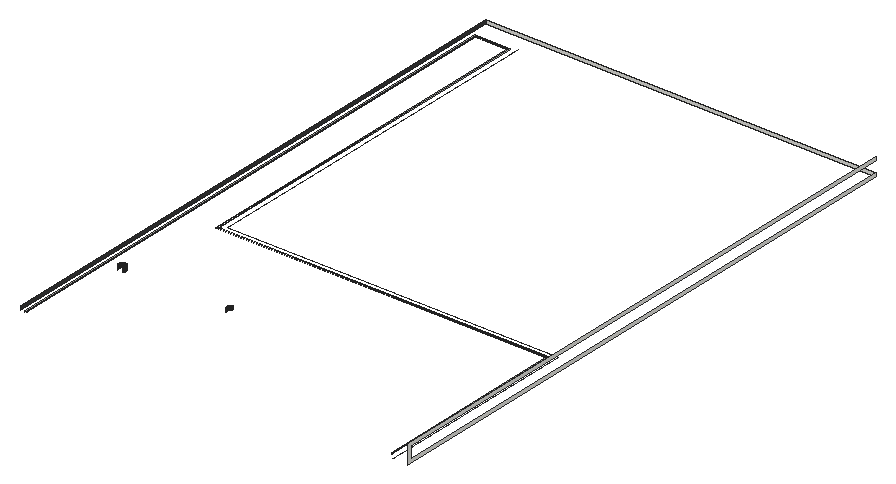
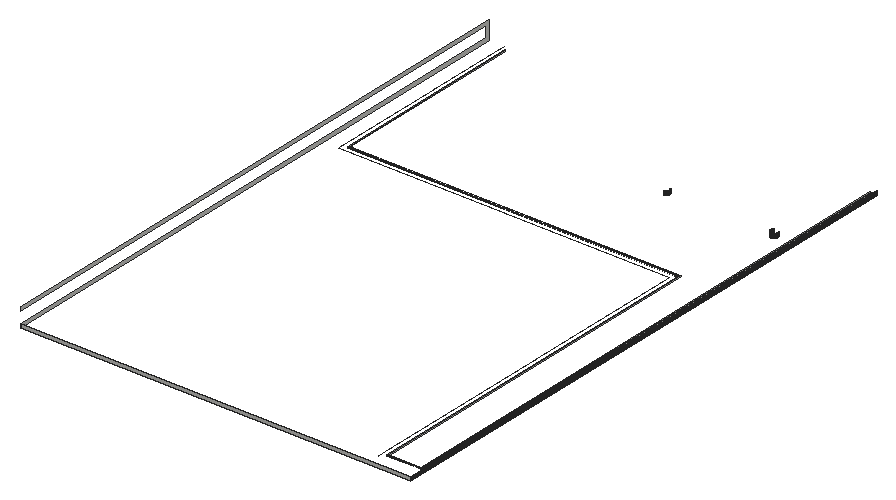
# SketchUp Ruby script. Lengths in inches.
U = 1.inch
M = Sketchup.active_model
def pt(a) = Geom::Point3d.new(a.map { |v| v * U })
def face(e, loops, mat)
  f = e.add_face(loops[0].map { |a| pt(a) })
  loops[1..].each { |l| e.add_face(l.map { |a| pt(a) }).erase! }
  f.material = f.back_material = mat if mat
  f
end
# faces: each face lists its corners as indices into pts; further lists are holes
def faces(e, pts, list, mat = nil) = list.each { |f| face(e, (f[0].is_a?(Array) ? f : [f]).map { |l| l.map { |i| pts[i] } }, mat) }
# xy, xz, yz: faces in a plane at the given z, y or x. An outline is a flat list of corners, or four numbers for a rectangle; further outlines are holes
def ring(l) = l.size == 4 ? [[l[0], l[1]], [l[2], l[1]], [l[2], l[3]], [l[0], l[3]]] : l.each_slice(2).to_a
def flat(e, list, mat, &to3) = list.each { |f| face(e, (f[0].is_a?(Array) ? f : [f]).map { |l| ring(l).map { |u, v| to3.(u, v) } }, mat) }
def xy(e, z, list, mat = nil) = flat(e, list, mat) { |x, y| [x, y, z] }
def xz(e, y, list, mat = nil) = flat(e, list, mat) { |x, z| [x, y, z] }
def yz(e, x, list, mat = nil) = flat(e, list, mat) { |y, z| [x, y, z] }
def lines(e, pts, list) = list.each { |a, b| e.add_line(pt(pts[a]), pt(pts[b])) }
# prism: a flat outline (further loops are holes) pulled along v
def prism(e, loops, v, mat = nil)
  f = face(e, loops, mat); d = Geom::Vector3d.new(v.map { |x| x * U })
  f.pushpull(f.normal.samedirection?(d) ? d.length : -d.length)
end
def box(e, o, s, mat = nil) = prism(e, [[o, [o[0] + s[0], o[1], o[2]], [o[0] + s[0], o[1] + s[1], o[2]], [o[0], o[1] + s[1], o[2]]]], [0, 0, s[2]], mat)
def at(x, y, z, deg = 0) = Geom::Transformation.translation(pt([x, y, z])) * Geom::Transformation.rotation(ORIGIN, Z_AXIS, deg.degrees)
def axes(o, x, y, z) = Geom::Transformation.new([*x, 0, *y, 0, *z, 0, *pt(o).to_a, 1])
def part(name) = M.definitions.add(name)
# library, detail: a bought-in or finely detailed component or shape, given as its bounding box
def library(name, o, s) = part(name).tap { |d| box(d.entities, o, s) }
def detail(e, o, s) = box(e.add_group.entities, o, s)
def put(e, d, t, mat = nil) = e.add_instance(d, t).tap { |i| i.material = mat if mat }
def group(e, t, mat = nil) = e.add_group.tap { |g| g.transformation = t; g.material = mat if mat }.entities
root = M.entities
M.materials.add("1496 AP 8293 CARBON COPY").color = [58, 58, 58]
xz(root,180.5,[[28.84,258,28.92,261],[28.92,258,29,261],[29,258,29.08,261],[29.08,258,29.16,261]])
xz(root,256,[[42,258,309,258.5]])
xz(root,257,[[43,258,310,258.5]])
xz(root,550,[[16,258,42,258.5]])
xz(root,551,[[15,258,43,258.5]])
xz(root,567,[[11,258,326,261]])
yz(root,11,[[97,258,567,261]],"1496 AP 8293 CARBON COPY")
yz(root,15,[[97,258,551,258.5]])
yz(root,16,[[97,258,550,258.5]])
yz(root,26,[[177.34,258,177.42,261],[177.42,258,177.5,261],[177.5,258,177.58,261],[177.58,258,177.66,261]])
yz(root,32,[[177.34,258,177.42,261],[177.42,258,177.5,261],[177.5,258,177.58,261],[177.58,258,177.66,261]])
yz(root,42,[[256,258,550,258.5]])
yz(root,43,[[257,258,551,258.5]])
yz(root,113.67,[[177.34,258,177.42,261],[177.42,258,177.5,261],[177.5,258,177.58,261],[177.58,258,177.66,261]])
yz(root,113.68,[[177.1875,258,177.26,261],[177.74,258,177.8125,261]])
yz(root,309,[[99,258,256,258.5]])
yz(root,310,[[98,258,257,258.5]])
yz(root,326,[[94,258,567,258,567,261,97,261,97,270,567,270,567,273,94,273]])
p = [[26.67,175.61,258],[26.62,175.67,258],[26.62,175.67,261],[26.67,175.61,261],[31.33,175.61,258],[31.28,175.55,258],
  [31.28,175.55,261],[31.33,175.61,261],[31.38,175.67,258],[31.38,175.67,261],[114.39,175.55,258],[114.34,175.61,258],
  [114.34,175.61,261],[114.39,175.55,261],[114.29,175.67,258],[114.29,175.67,261],[26.57,175.74,258],[26.53,175.8,258],
  [26.53,175.8,261],[26.57,175.74,261],[31.43,175.74,258],[31.43,175.74,261],[31.47,175.8,258],[31.47,175.8,261],
  [114.24,175.74,258],[114.24,175.74,261],[114.19,175.8,258],[114.19,175.8,261],[26.48,175.87,258],[26.48,175.87,261],
  [31.52,175.87,258],[31.52,175.87,261],[114.15,175.87,258],[114.15,175.87,261],[26.44,175.93,258],[26.44,175.93,261],
  [26.4,176,258],[26.4,176,261],[31.56,175.93,258],[31.56,175.93,261],[31.6,176,258],[31.6,176,261],
  [114.11,175.93,258],[114.11,175.93,261],[114.07,176,258],[114.07,176,261],[26.36,176.07,258],[26.36,176.07,261],
  [31.64,176.07,258],[31.64,176.07,261],[114.03,176.07,258],[114.03,176.07,261],[26.33,176.14,258],[26.33,176.14,261],
  [26.29,176.21,258],[26.29,176.21,261],[31.67,176.14,258],[31.67,176.14,261],[31.71,176.21,258],[31.71,176.21,261],
  [113.99,176.14,258],[113.99,176.14,261],[113.96,176.21,258],[113.96,176.21,261],[26.26,176.28,258],[26.26,176.28,261],
  [31.74,176.28,258],[31.74,176.28,261],[113.93,176.28,258],[113.93,176.28,261],[26.23,176.35,258],[26.23,176.35,261],
  [31.77,176.35,258],[31.77,176.35,261],[113.9,176.35,258],[113.9,176.35,261],[26.2,176.42,258],[26.2,176.42,261],
  [26.17,176.5,258],[26.17,176.5,261],[31.8,176.42,258],[31.8,176.42,261],[31.83,176.5,258],[31.83,176.5,261],
  [113.87,176.42,258],[113.84,176.5,258],[113.84,176.5,261],[113.87,176.42,261],[26.15,176.57,258],[26.15,176.57,261],
  [31.85,176.57,258],[31.85,176.57,261],[113.8125,176.57,258],[113.8125,176.57,261],[26.125,176.65,258],[26.125,176.65,261],
  [26.1,176.72,258],[26.1,176.72,261],[31.875,176.65,258],[31.875,176.65,261],[31.9,176.72,258],[31.9,176.72,261],
  [113.79,176.65,258],[113.79,176.65,261],[113.77,176.72,258],[113.77,176.72,261],[26.08,176.8,258],[26.08,176.8,261],
  [31.92,176.8,258],[31.92,176.8,261],[113.75,176.8,258],[113.75,176.8,261],[26.07,176.875,258],[26.07,176.875,261],
  [31.93,176.875,258],[31.93,176.875,261],[113.73,176.875,258],[113.73,176.875,261],[26.05,176.95,258],[26.05,176.95,261],
  [31.95,176.95,258],[31.95,176.95,261],[113.72,176.95,258],[113.72,176.95,261],[26.04,177.03,258],[26.04,177.03,261],
  [26.03,177.11,258],[26.03,177.11,261],[31.96,177.03,258],[31.96,177.03,261],[31.97,177.11,258],[31.97,177.11,261],
  [113.7,177.03,258],[113.7,177.03,261],[113.69,177.11,258],[113.69,177.11,261],[26.02,177.1875,258],[26.02,177.1875,261],
  [31.98,177.1875,258],[31.98,177.1875,261],[113.68,177.1875,258],[113.68,177.1875,261],[26.01,177.26,258],[26.01,177.26,261],
  [31.99,177.26,258],[31.99,177.26,261],[26,177.34,258],[26,177.34,261],[32,177.34,258],[32,177.34,261],
  [113.68,177.26,258],[113.67,177.34,258],[113.67,177.34,261],[113.68,177.26,261],[26,177.66,258],[26.01,177.74,258],
  [26.01,177.74,261],[26,177.66,261],[26.02,177.8125,258],[26.02,177.8125,261],[31.99,177.74,258],[32,177.66,258],
  [32,177.66,261],[31.99,177.74,261],[31.98,177.8125,258],[31.98,177.8125,261],[113.67,177.66,258],[113.68,177.74,258],
  [113.68,177.74,261],[113.67,177.66,261],[26.03,177.89,258],[26.03,177.89,261],[31.97,177.89,258],[31.97,177.89,261],
  [113.68,177.8125,258],[113.69,177.89,258],[113.69,177.89,261],[113.68,177.8125,261],[26.04,177.97,258],[26.04,177.97,261],
  [31.96,177.97,258],[31.96,177.97,261],[113.7,177.97,258],[113.7,177.97,261],[26.05,178.05,258],[26.05,178.05,261],
  [26.07,178.125,258],[26.07,178.125,261],[31.95,178.05,258],[31.95,178.05,261],[31.93,178.125,258],[31.93,178.125,261],
  [113.72,178.05,258],[113.72,178.05,261],[113.73,178.125,258],[113.73,178.125,261],[26.08,178.2,258],[26.08,178.2,261],
  [31.92,178.2,258],[31.92,178.2,261],[113.75,178.2,258],[113.75,178.2,261],[26.1,178.28,258],[26.1,178.28,261],
  [31.9,178.28,258],[31.9,178.28,261],[113.77,178.28,258],[113.77,178.28,261],[26.125,178.35,258],[26.125,178.35,261],
  [31.875,178.35,258],[31.875,178.35,261],[113.79,178.35,258],[113.79,178.35,261],[26.15,178.43,258],[26.15,178.43,261],
  [26.17,178.5,258],[26.17,178.5,261],[31.83,178.5,258],[31.85,178.43,258],[31.85,178.43,261],[31.83,178.5,261],
  [113.8125,178.43,258],[113.8125,178.43,261],[113.84,178.5,258],[113.84,178.5,261],[26.2,178.58,258],[26.2,178.58,261],
  [31.8,178.58,258],[31.8,178.58,261],[113.87,178.58,258],[113.87,178.58,261],[26.23,178.65,258],[26.23,178.65,261],
  [26.26,178.72,258],[26.26,178.72,261],[31.74,178.72,258],[31.77,178.65,258],[31.77,178.65,261],[31.74,178.72,261],
  [113.9,178.65,258],[113.9,178.65,261],[113.93,178.72,258],[113.93,178.72,261],[26.29,178.79,258],[26.29,178.79,261],
  [31.71,178.79,258],[31.71,178.79,261],[113.96,178.79,258],[113.96,178.79,261],[26.33,178.86,258],[26.33,178.86,261],
  [31.67,178.86,258],[31.67,178.86,261],[113.99,178.86,258],[113.99,178.86,261],[26.36,178.93,258],[26.36,178.93,261],
  [26.4,179,258],[26.4,179,261],[31.64,178.93,258],[31.64,178.93,261],[31.6,179,258],[31.6,179,261],
  [114.03,178.93,258],[114.03,178.93,261],[114.07,179,258],[114.07,179,261],[26.44,179.07,258],[26.44,179.07,261],
  [31.56,179.07,258],[31.56,179.07,261],[114.11,179.07,258],[114.11,179.07,261],[26.48,179.13,258],[26.48,179.13,261],
  [26.53,179.2,258],[26.53,179.2,261],[31.52,179.13,258],[31.52,179.13,261],[31.47,179.2,258],[31.47,179.2,261],
  [114.15,179.13,258],[114.15,179.13,261],[114.19,179.2,258],[114.19,179.2,261],[26.57,179.26,258],[26.57,179.26,261],
  [31.43,179.26,258],[31.43,179.26,261],[114.24,179.26,258],[114.24,179.26,261],[26.62,179.33,258],[26.62,179.33,261],
  [26.67,179.39,258],[26.67,179.39,261],[31.33,179.39,258],[31.38,179.33,258],[31.38,179.33,261],[31.33,179.39,261],
  [114.29,179.33,258],[114.29,179.33,261],[114.34,179.39,258],[114.34,179.39,261],[26.72,179.45,258],[26.72,179.45,261],
  [26.77,179.51,258],[26.77,179.51,261],[31.23,179.51,258],[31.28,179.45,258],[31.28,179.45,261],[31.23,179.51,261],
  [114.39,179.45,258],[114.39,179.45,261],[114.4375,179.51,258],[114.4375,179.51,261],[26.82,179.57,258],[26.82,179.57,261],
  [31.18,179.57,258],[31.18,179.57,261],[114.49,179.57,258],[114.49,179.57,261],[26.88,179.62,258],[26.88,179.62,261],
  [26.93,179.68,258],[26.93,179.68,261],[31.12,179.62,258],[31.12,179.62,261],[31.07,179.68,258],[31.07,179.68,261],
  [114.55,179.62,258],[114.55,179.62,261],[114.6,179.68,258],[114.6,179.68,261],[26.99,179.73,258],[26.99,179.73,261],
  [27.05,179.78,258],[27.05,179.78,261],[30.95,179.78,258],[31.01,179.73,258],[31.01,179.73,261],[30.95,179.78,261],
  [114.66,179.73,258],[114.66,179.73,261],[114.72,179.78,258],[114.72,179.78,261],[27.11,179.83,258],[27.11,179.83,261],
  [27.17,179.88,258],[27.17,179.88,261],[30.83,179.88,258],[30.89,179.83,258],[30.89,179.83,261],[30.83,179.88,261],
  [114.78,179.83,258],[114.78,179.83,261],[114.84,179.88,258],[114.84,179.88,261],[27.24,179.93,258],[27.24,179.93,261],
  [27.3,179.97,258],[27.3,179.97,261],[30.7,179.97,258],[30.76,179.93,258],[30.76,179.93,261],[30.7,179.97,261],
  [114.9,179.93,258],[114.9,179.93,261],[114.97,179.97,258],[114.97,179.97,261],[27.37,180.02,258],[27.37,180.02,261],
  [27.43,180.06,258],[27.43,180.06,261],[30.63,180.02,258],[30.63,180.02,261],[30.57,180.06,258],[30.57,180.06,261],
  [115.03,180.02,258],[115.03,180.02,261],[115.1,180.06,258],[115.1,180.06,261],[27.5,180.1,258],[27.5,180.1,261],
  [27.57,180.14,258],[27.57,180.14,261],[27.64,180.17,258],[27.64,180.17,261],[30.43,180.14,258],[30.5,180.1,258],
  [30.5,180.1,261],[30.43,180.14,261],[30.36,180.17,258],[30.36,180.17,261],[115.17,180.1,258],[115.17,180.1,261],
  [115.24,180.14,258],[115.24,180.14,261],[115.3,180.17,258],[115.3,180.17,261],[27.71,180.21,258],[27.71,180.21,261],
  [27.78,180.24,258],[27.78,180.24,261],[27.85,180.27,258],[27.85,180.27,261],[30.15,180.27,258],[30.22,180.24,258],
  [30.22,180.24,261],[30.15,180.27,261],[30.29,180.21,258],[30.29,180.21,261],[115.375,180.21,258],[115.375,180.21,261],
  [115.45,180.24,258],[115.45,180.24,261],[115.52,180.27,258],[115.52,180.27,261],[27.92,180.3,258],[27.92,180.3,261],
  [28,180.33,258],[28,180.33,261],[28.07,180.35,258],[28.07,180.35,261],[29.93,180.35,258],[30,180.33,258],
  [30,180.33,261],[29.93,180.35,261],[30.08,180.3,258],[30.08,180.3,261],[115.59,180.3,258],[115.59,180.3,261],
  [115.67,180.33,258],[115.67,180.33,261],[115.74,180.35,258],[115.74,180.35,261],[28.15,180.375,258],[28.15,180.375,261],
  [28.22,180.4,258],[28.22,180.4,261],[28.3,180.42,258],[28.3,180.42,261],[28.375,180.43,258],[28.375,180.43,261],
  [28.45,180.45,258],[28.45,180.45,261],[28.53,180.46,258],[28.53,180.46,261],[29.55,180.45,258],[29.625,180.43,258],
  [29.625,180.43,261],[29.55,180.45,261],[29.47,180.46,258],[29.47,180.46,261],[29.7,180.42,258],[29.7,180.42,261],
  [29.78,180.4,258],[29.78,180.4,261],[29.85,180.375,258],[29.85,180.375,261],[115.81,180.375,258],[115.81,180.375,261],
  [115.89,180.4,258],[115.89,180.4,261],[115.97,180.42,258],[115.97,180.42,261],[116.04,180.43,258],[116.04,180.43,261],
  [28.61,180.47,258],[28.61,180.47,261],[28.6875,180.48,258],[28.6875,180.48,261],[28.76,180.49,258],[28.76,180.49,261],
  [28.84,180.5,258],[28.84,180.5,261],[29.24,180.49,258],[29.3125,180.48,258],[29.3125,180.48,261],[29.24,180.49,261],
  [29.16,180.5,258],[29.16,180.5,261],[29.39,180.47,258],[29.39,180.47,261],[47,555,258],[47,261,258],
  [314,261,258],[314,94,258]]
faces(root,p,[[0,1,2,3],[4,5,6,7],[8,4,7,9],[10,11,12,13],[11,14,15,12],[16,17,18,19],[1,16,19,2],[20,8,9,21],
  [22,20,21,23],[14,24,25,15],[24,26,27,25],[17,28,29,18],[30,22,23,31],[26,32,33,27],[28,34,35,29],[34,36,37,35],
  [38,30,31,39],[40,38,39,41],[32,42,43,33],[42,44,45,43],[36,46,47,37],[48,40,41,49],[44,50,51,45],[46,52,53,47],
  [52,54,55,53],[56,48,49,57],[58,56,57,59],[50,60,61,51],[60,62,63,61],[54,64,65,55],[66,58,59,67],[62,68,69,63],
  [64,70,71,65],[72,66,67,73],[68,74,75,69],[70,76,77,71],[76,78,79,77],[80,72,73,81],[82,80,81,83],[84,85,86,87],
  [74,84,87,75],[78,88,89,79],[90,82,83,91],[85,92,93,86],[88,94,95,89],[94,96,97,95],[98,90,91,99],[100,98,99,101],
  [92,102,103,93],[102,104,105,103],[96,106,107,97],[108,100,101,109],[104,110,111,105],[106,112,113,107],[114,108,109,115],[110,116,117,111],
  [112,118,119,113],[120,114,115,121],[116,122,123,117],[118,124,125,119],[124,126,127,125],[128,120,121,129],[130,128,129,131],[122,132,133,123],
  [132,134,135,133],[126,136,137,127],[138,130,131,139],[134,140,141,135],[136,142,143,137],[144,138,139,145],[142,146,147,143],[148,144,145,149],
  [150,151,152,153],[154,155,156,157],[155,158,159,156],[160,161,162,163],[164,160,163,165],[166,167,168,169],[158,170,171,159],[172,164,165,173],
  [174,175,176,177],[170,178,179,171],[180,172,173,181],[175,182,183,176],[178,184,185,179],[184,186,187,185],[188,180,181,189],[190,188,189,191],
  [182,192,193,183],[192,194,195,193],[186,196,197,187],[198,190,191,199],[194,200,201,195],[196,202,203,197],[204,198,199,205],[200,206,207,201],
  [202,208,209,203],[210,204,205,211],[206,212,213,207],[208,214,215,209],[214,216,217,215],[218,219,220,221],[219,210,211,220],[212,222,223,213],
  [222,224,225,223],[216,226,227,217],[228,218,221,229],[224,230,231,225],[226,232,233,227],[232,234,235,233],[236,237,238,239],[237,228,229,238],
  [230,240,241,231],[240,242,243,241],[234,244,245,235],[246,236,239,247],[242,248,249,243],[244,250,251,245],[252,246,247,253],[248,254,255,249],
  [250,256,257,251],[256,258,259,257],[260,252,253,261],[262,260,261,263],[254,264,265,255],[264,266,267,265],[258,268,269,259],[270,262,263,271],
  [266,272,273,267],[268,274,275,269],[274,276,277,275],[278,270,271,279],[280,278,279,281],[272,282,283,273],[282,284,285,283],[276,286,287,277],
  [288,280,281,289],[284,290,291,285],[286,292,293,287],[292,294,295,293],[296,297,298,299],[297,288,289,298],[290,300,301,291],[300,302,303,301],
  [294,304,305,295],[304,306,307,305],[308,309,310,311],[309,296,299,310],[302,312,313,303],[312,314,315,313],[306,316,317,307],[318,308,311,319],
  [314,320,321,315],[316,322,323,317],[322,324,325,323],[326,318,319,327],[328,326,327,329],[320,330,331,321],[330,332,333,331],[324,334,335,325],
  [334,336,337,335],[338,339,340,341],[339,328,329,340],[332,342,343,333],[342,344,345,343],[336,346,347,337],[346,348,349,347],[350,351,352,353],
  [351,338,341,352],[344,354,355,345],[354,356,357,355],[348,358,359,349],[358,360,361,359],[362,363,364,365],[363,350,353,364],[356,366,367,357],
  [366,368,369,367],[360,370,371,361],[370,372,373,371],[374,362,365,375],[376,374,375,377],[368,378,379,369],[378,380,381,379],[372,382,383,373],
  [382,384,385,383],[384,386,387,385],[388,389,390,391],[392,388,391,393],[389,376,377,390],[380,394,395,381],[394,396,397,395],[396,398,399,397],
  [386,400,401,387],[400,402,403,401],[402,404,405,403],[406,407,408,409],[407,410,411,408],[410,392,393,411],[398,412,413,399],[412,414,415,413],
  [414,416,417,415],[404,418,419,405],[418,420,421,419],[420,422,423,421],[424,425,426,427],[425,428,429,426],[428,406,409,429],[416,430,431,417],
  [430,432,433,431],[432,434,435,433],[422,436,437,423],[436,438,439,437],[438,440,441,439],[440,442,443,441],[442,444,445,443],[444,446,447,445],
  [448,449,450,451],[452,448,451,453],[449,454,455,450],[454,456,457,455],[456,458,459,457],[458,424,427,459],[434,460,461,435],[460,462,463,461],
  [462,464,465,463],[464,466,467,465],[446,468,469,447],[468,470,471,469],[470,472,473,471],[472,474,475,473],[476,477,478,479],[480,476,479,481],
  [477,482,483,478],[482,452,453,483]])
lines(root,p,[[484,485],[485,486],[486,487]])
